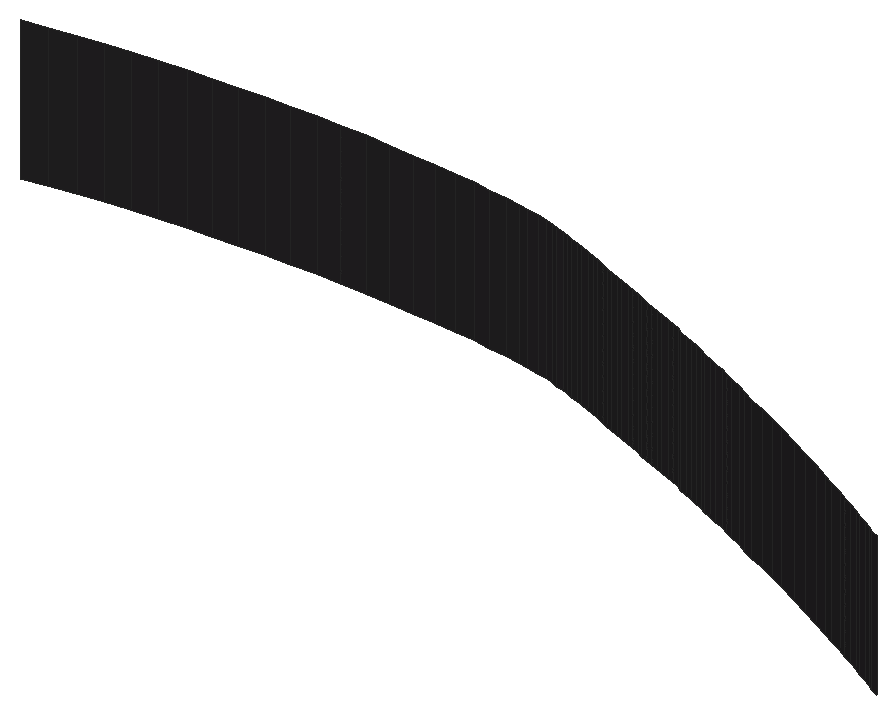
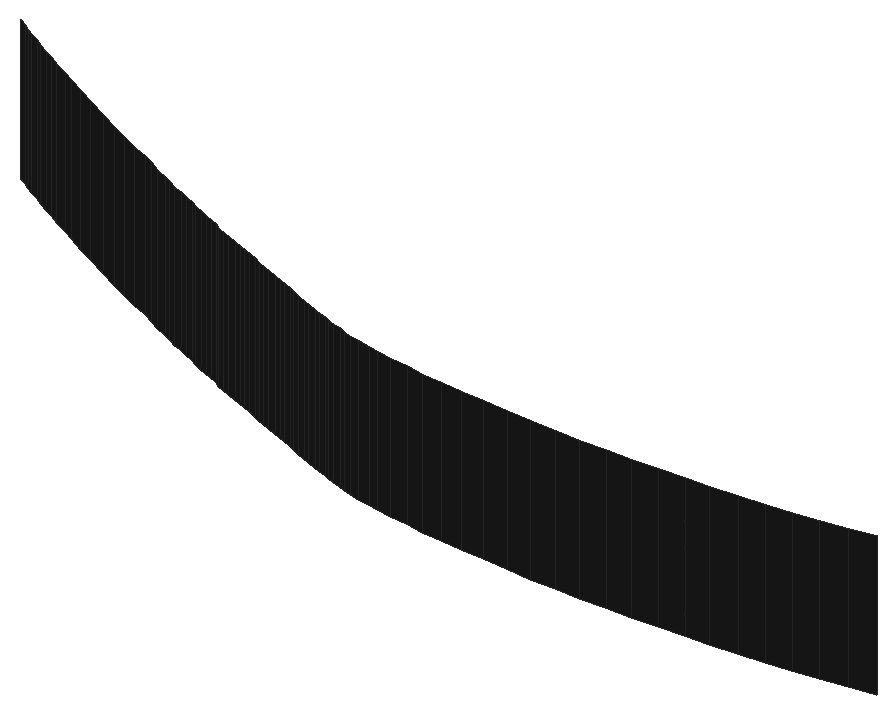
# SketchUp Ruby script. Lengths in inches.
U = 1.inch
M = Sketchup.active_model
def pt(a) = Geom::Point3d.new(a.map { |v| v * U })
def face(e, loops, mat)
  f = e.add_face(loops[0].map { |a| pt(a) })
  loops[1..].each { |l| e.add_face(l.map { |a| pt(a) }).erase! }
  f.material = f.back_material = mat if mat
  f
end
# faces: each face lists its corners as indices into pts; further lists are holes
def faces(e, pts, list, mat = nil) = list.each { |f| face(e, (f[0].is_a?(Array) ? f : [f]).map { |l| l.map { |i| pts[i] } }, mat) }
# xy, xz, yz: faces in a plane at the given z, y or x. An outline is a flat list of corners, or four numbers for a rectangle; further outlines are holes
def ring(l) = l.size == 4 ? [[l[0], l[1]], [l[2], l[1]], [l[2], l[3]], [l[0], l[3]]] : l.each_slice(2).to_a
def flat(e, list, mat, &to3) = list.each { |f| face(e, (f[0].is_a?(Array) ? f : [f]).map { |l| ring(l).map { |u, v| to3.(u, v) } }, mat) }
def xy(e, z, list, mat = nil) = flat(e, list, mat) { |x, y| [x, y, z] }
def xz(e, y, list, mat = nil) = flat(e, list, mat) { |x, z| [x, y, z] }
def yz(e, x, list, mat = nil) = flat(e, list, mat) { |y, z| [x, y, z] }
def lines(e, pts, list) = list.each { |a, b| e.add_line(pt(pts[a]), pt(pts[b])) }
# prism: a flat outline (further loops are holes) pulled along v
def prism(e, loops, v, mat = nil)
  f = face(e, loops, mat); d = Geom::Vector3d.new(v.map { |x| x * U })
  f.pushpull(f.normal.samedirection?(d) ? d.length : -d.length)
end
def box(e, o, s, mat = nil) = prism(e, [[o, [o[0] + s[0], o[1], o[2]], [o[0] + s[0], o[1] + s[1], o[2]], [o[0], o[1] + s[1], o[2]]]], [0, 0, s[2]], mat)
def at(x, y, z, deg = 0) = Geom::Transformation.translation(pt([x, y, z])) * Geom::Transformation.rotation(ORIGIN, Z_AXIS, deg.degrees)
def axes(o, x, y, z) = Geom::Transformation.new([*x, 0, *y, 0, *z, 0, *pt(o).to_a, 1])
def part(name) = M.definitions.add(name)
# library, detail: a bought-in or finely detailed component or shape, given as its bounding box
def library(name, o, s) = part(name).tap { |d| box(d.entities, o, s) }
def detail(e, o, s) = box(e.add_group.entities, o, s)
def put(e, d, t, mat = nil) = e.add_instance(d, t).tap { |i| i.material = mat if mat }
def group(e, t, mat = nil) = e.add_group.tap { |g| g.transformation = t; g.material = mat if mat }.entities
root = M.entities
M.materials.add("Marble_07_1K").color = [36, 34, 36]
xz(root,776.63,[[334.73,18,334.91,19]],"Marble_07_1K")
xz(root,776.64,[[335.09,18,335.26,19],[335.26,18,335.4375,19]],"Marble_07_1K")
p = [[340.3,774.96,18],[340.35,774.93,18],[340.35,774.93,19],[340.3,774.96,19],[340.4,774.9,18],[340.4,774.9,19],
  [340.45,774.875,18],[340.45,774.875,19],[340.12,775.06,18],[340.18,775.03,18],[340.18,775.03,19],[340.12,775.06,19],
  [340.24,774.99,18],[340.24,774.99,19],[339.89,775.18,18],[339.98,775.14,18],[339.98,775.14,19],[339.89,775.18,19],
  [340.05,775.1,18],[340.05,775.1,19],[339.69,775.29,18],[339.8,775.23,18],[339.8,775.23,19],[339.69,775.29,19],
  [339.43,775.42,18],[339.57,775.35,18],[339.57,775.35,19],[339.43,775.42,19],[339.29,775.49,18],[339.29,775.49,19],
  [339.06,775.6,18],[339.17,775.55,18],[339.17,775.55,19],[339.06,775.6,19],[338.88,775.68,18],[338.96,775.64,18],
  [338.96,775.64,19],[338.88,775.68,19],[338.73,775.75,18],[338.8,775.72,18],[338.8,775.72,19],[338.73,775.75,19],
  [338.49,775.86,18],[338.55,775.83,18],[338.55,775.83,19],[338.49,775.86,19],[338.61,775.81,18],[338.61,775.81,19],
  [338.67,775.78,18],[338.67,775.78,19],[338.28,775.95,18],[338.33,775.93,18],[338.33,775.93,19],[338.28,775.95,19],
  [338.38,775.91,18],[338.38,775.91,19],[338.4375,775.88,18],[338.4375,775.88,19],[338.03,776.06,18],[338.08,776.04,18],
  [338.08,776.04,19],[338.03,776.06,19],[338.13,776.02,18],[338.13,776.02,19],[338.18,775.99,18],[338.18,775.99,19],
  [338.23,775.97,18],[338.23,775.97,19],[337.77,776.16,18],[337.82,776.14,18],[337.82,776.14,19],[337.77,776.16,19],
  [337.87,776.12,18],[337.87,776.12,19],[337.92,776.1,18],[337.92,776.1,19],[337.97,776.08,18],[337.97,776.08,19],
  [337.51,776.26,18],[337.56,776.24,18],[337.56,776.24,19],[337.51,776.26,19],[337.62,776.22,18],[337.62,776.22,19],
  [337.67,776.2,18],[337.67,776.2,19],[337.72,776.18,18],[337.72,776.18,19],[337.26,776.36,18],[337.31,776.34,18],
  [337.31,776.34,19],[337.26,776.36,19],[337.36,776.32,18],[337.36,776.32,19],[337.41,776.3,18],[337.41,776.3,19],
  [337.46,776.28,18],[337.46,776.28,19],[337.01,776.45,18],[337.06,776.43,18],[337.06,776.43,19],[337.01,776.45,19],
  [337.1,776.42,18],[337.1,776.42,19],[337.15,776.4,18],[337.15,776.4,19],[337.21,776.38,18],[337.21,776.38,19],
  [333.14,776.46,18],[333.3125,776.49,18],[333.3125,776.49,19],[333.14,776.46,19],[333.49,776.52,18],[333.49,776.52,19],
  [333.67,776.54,18],[333.67,776.54,19],[333.84,776.5625,18],[333.84,776.5625,19],[336.58,776.56,18],[336.66,776.54,18],
  [336.66,776.54,19],[336.58,776.56,19],[336.74,776.53,18],[336.74,776.53,19],[336.8,776.52,18],[336.8,776.52,19],
  [336.86,776.5,18],[336.86,776.5,19],[336.91,776.48,18],[336.91,776.48,19],[336.96,776.47,18],[336.96,776.47,19],
  [334.02,776.58,18],[334.02,776.58,19],[334.2,776.6,18],[334.2,776.6,19],[334.375,776.61,18],[334.375,776.61,19],
  [334.55,776.62,18],[334.55,776.62,19],[334.73,776.63,18],[334.73,776.63,19],[334.91,776.63,18],[335.09,776.64,18],
  [335.09,776.64,19],[334.91,776.63,19],[335.4375,776.64,18],[335.61,776.63,18],[335.61,776.63,19],[335.4375,776.64,19],
  [335.78,776.625,18],[335.78,776.625,19],[335.9375,776.62,18],[335.9375,776.62,19],[336.09,776.61,18],[336.09,776.61,19],
  [336.23,776.6,18],[336.23,776.6,19],[336.36,776.58,18],[336.36,776.58,19],[336.48,776.57,18],[336.48,776.57,19]]
faces(root,p,[[0,1,2,3],[1,4,5,2],[4,6,7,5],[8,9,10,11],[9,12,13,10],[12,0,3,13],[14,15,16,17],[15,18,19,16],
  [18,8,11,19],[20,21,22,23],[21,14,17,22],[24,25,26,27],[25,20,23,26],[28,24,27,29],[30,31,32,33],[31,28,29,32],
  [34,35,36,37],[35,30,33,36],[38,39,40,41],[39,34,37,40],[42,43,44,45],[43,46,47,44],[46,48,49,47],[48,38,41,49],
  [50,51,52,53],[51,54,55,52],[54,56,57,55],[56,42,45,57],[58,59,60,61],[59,62,63,60],[62,64,65,63],[64,66,67,65],
  [66,50,53,67],[68,69,70,71],[69,72,73,70],[72,74,75,73],[74,76,77,75],[76,58,61,77],[78,79,80,81],[79,82,83,80],
  [82,84,85,83],[84,86,87,85],[86,68,71,87],[88,89,90,91],[89,92,93,90],[92,94,95,93],[94,96,97,95],[96,78,81,97],
  [98,99,100,101],[99,102,103,100],[102,104,105,103],[104,106,107,105],[106,88,91,107],[108,109,110,111],[109,112,113,110],[112,114,115,113],
  [114,116,117,115],[118,119,120,121],[119,122,123,120],[122,124,125,123],[124,126,127,125],[126,128,129,127],[128,130,131,129],[130,98,101,131],
  [116,132,133,117],[132,134,135,133],[134,136,137,135],[136,138,139,137],[138,140,141,139],[142,143,144,145],[146,147,148,149],[147,150,151,148],
  [150,152,153,151],[152,154,155,153],[154,156,157,155],[156,158,159,157],[158,160,161,159],[160,118,121,161]],"Marble_07_1K")
